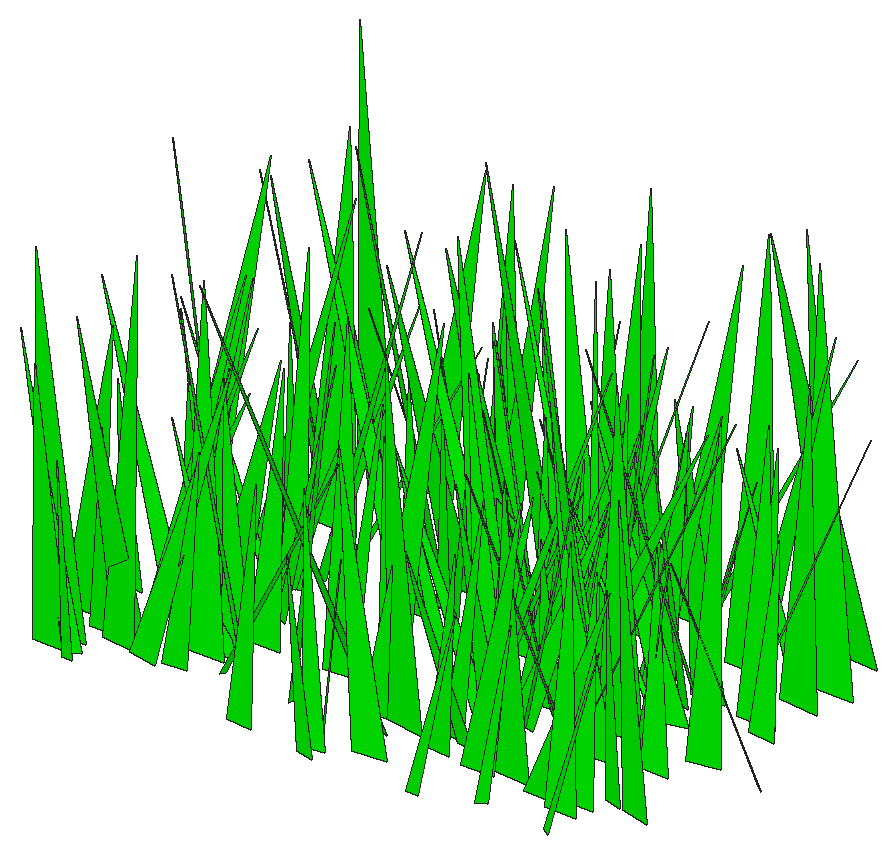
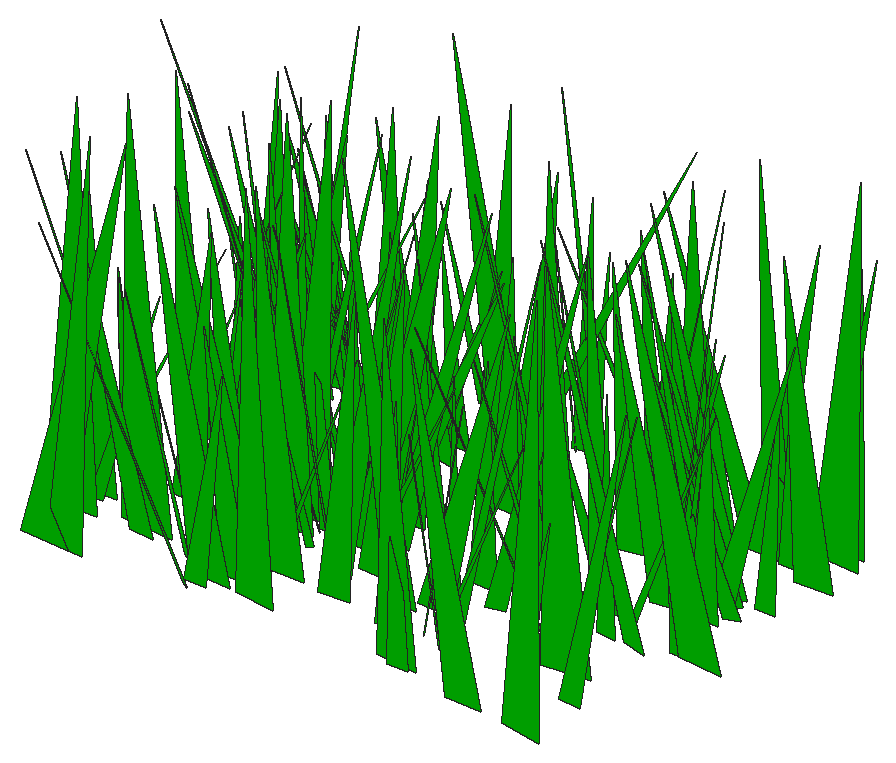
# SketchUp Ruby script. Lengths in inches.
U = 1.inch
M = Sketchup.active_model
def pt(a) = Geom::Point3d.new(a.map { |v| v * U })
def face(e, loops, mat)
  f = e.add_face(loops[0].map { |a| pt(a) })
  loops[1..].each { |l| e.add_face(l.map { |a| pt(a) }).erase! }
  f.material = f.back_material = mat if mat
  f
end
# faces: each face lists its corners as indices into pts; further lists are holes
def faces(e, pts, list, mat = nil) = list.each { |f| face(e, (f[0].is_a?(Array) ? f : [f]).map { |l| l.map { |i| pts[i] } }, mat) }
# xy, xz, yz: faces in a plane at the given z, y or x. An outline is a flat list of corners, or four numbers for a rectangle; further outlines are holes
def ring(l) = l.size == 4 ? [[l[0], l[1]], [l[2], l[1]], [l[2], l[3]], [l[0], l[3]]] : l.each_slice(2).to_a
def flat(e, list, mat, &to3) = list.each { |f| face(e, (f[0].is_a?(Array) ? f : [f]).map { |l| ring(l).map { |u, v| to3.(u, v) } }, mat) }
def xy(e, z, list, mat = nil) = flat(e, list, mat) { |x, y| [x, y, z] }
def xz(e, y, list, mat = nil) = flat(e, list, mat) { |x, z| [x, y, z] }
def yz(e, x, list, mat = nil) = flat(e, list, mat) { |y, z| [x, y, z] }
def lines(e, pts, list) = list.each { |a, b| e.add_line(pt(pts[a]), pt(pts[b])) }
# prism: a flat outline (further loops are holes) pulled along v
def prism(e, loops, v, mat = nil)
  f = face(e, loops, mat); d = Geom::Vector3d.new(v.map { |x| x * U })
  f.pushpull(f.normal.samedirection?(d) ? d.length : -d.length)
end
def box(e, o, s, mat = nil) = prism(e, [[o, [o[0] + s[0], o[1], o[2]], [o[0] + s[0], o[1] + s[1], o[2]], [o[0], o[1] + s[1], o[2]]]], [0, 0, s[2]], mat)
def at(x, y, z, deg = 0) = Geom::Transformation.translation(pt([x, y, z])) * Geom::Transformation.rotation(ORIGIN, Z_AXIS, deg.degrees)
def axes(o, x, y, z) = Geom::Transformation.new([*x, 0, *y, 0, *z, 0, *pt(o).to_a, 1])
def part(name) = M.definitions.add(name)
# library, detail: a bought-in or finely detailed component or shape, given as its bounding box
def library(name, o, s) = part(name).tap { |d| box(d.entities, o, s) }
def detail(e, o, s) = box(e.add_group.entities, o, s)
def put(e, d, t, mat = nil) = e.add_instance(d, t).tap { |i| i.material = mat if mat }
def group(e, t, mat = nil) = e.add_group.tap { |g| g.transformation = t; g.material = mat if mat }.entities
root = M.entities
M.materials.add("[0065_Lime]").color = [0, 255, 0]
c1 = part("fur_instance\#9")
p = [[0.8125,0,1.79],[0.67,-0.02,1.48],[0,-0.11,0],[0,0.11,0]]
faces(c1.entities,p,[[0,1,2,3]])
put(root,c1,axes([66.16,23.27,1.48],[-2.25498,-0.5227,0.91359],[3.79834,-0.33499,-0.21919],[0.81912,0.11443,3.53148]),"[0065_Lime]")
put(root,c1,axes([67.46,23.67,1.48],[-5.30338,0.46201,0.91212],[-3.37935,-0.75276,-0.22369],[0.8049,-0.11631,5.07068]),"[0065_Lime]")
put(root,c1,axes([66.42,19.65,1.48],[-0.43219,-1.1096,1.96187],[8.2532,-0.04828,0.28798],[-0.2379,0.34091,6.42628]),"[0065_Lime]")
put(root,c1,axes([67.59,30.83,1.48],[-6.41038,-0.13063,1.23017],[1.0527,-0.92088,0.35288],[1.4294,0.09238,5.257]),"[0065_Lime]")
put(root,c1,axes([67.24,31.19,1.48],[-4.99882,-0.57823,1.12049],[4.16598,-0.72211,-0.18998],[1.21459,0.09704,5.26315]),"[0065_Lime]")
put(root,c1,axes([67.28,19.06,1.48],[-5.88071,0.31736,1.53233],[-2.48222,-0.85299,-0.38313],[1.57741,-0.15913,5.10975]),"[0065_Lime]")
put(root,c1,axes([66.5,19.01,1.48],[-0.59034,-0.84096,1.06592],[6.12601,-0.08337,0.04076],[0.0776,0.18395,4.8915]),"[0065_Lime]")
put(root,c1,axes([65.95,21.25,1.48],[2.23254,-0.91834,0.53281],[6.56668,0.31413,-0.06238],[-0.13883,0.0906,5.61725]),"[0065_Lime]")
put(root,c1,axes([65.62,27.03,1.48],[4.08051,1.07997,0.77488],[-7.72236,0.57883,-0.12647],[-0.5848,-0.10791,7.07697]),"[0065_Lime]")
put(root,c1,axes([66.42,26.9,1.48],[1.95205,-0.53918,0.17976],[3.82124,0.276,0.28532],[-0.41291,0.00521,3.4902]),"[0065_Lime]")
put(root,c1,axes([67.27,33.47,1.48],[5.46045,0.90805,3.23613],[-7.03555,0.86389,-0.26824],[-2.84417,-0.39364,6.87649]),"[0065_Lime]")
put(root,c1,axes([67.94,25.54,1.48],[-8.50524,-0.12042,2.24811],[0.81591,-1.25665,-0.21315],[2.7762,0.00041,6.95004]),"[0065_Lime]")
put(root,c1,axes([68.75,26.39,1.48],[-5.34362,0.09829,0.51648],[-0.72094,-0.75548,-0.11765],[0.61046,-0.03187,4.38207]),"[0065_Lime]")
put(root,c1,axes([67.375,18.69,1.48],[-3.30569,-0.2481,1.3573],[2.08591,-0.49283,0.34268],[1.24527,0.16692,3.02907]),"[0065_Lime]")
put(root,c1,axes([67.18,20.69,1.48],[0.57871,-0.67566,0.21455],[4.81471,0.08189,0.04845],[-0.09074,0.03579,3.93909]),"[0065_Lime]")
put(root,c1,axes([67.29,24.75,1.48],[1.22999,-0.65895,0.25851],[4.68118,0.17589,0.28718],[-0.42265,0.03047,3.93303]),"[0065_Lime]")
put(root,c1,axes([68.31,20.53,1.48],[-3.34036,-0.8749,0.67141],[6.24904,-0.47614,-0.22049],[0.63043,0.084,5.74313]),"[0065_Lime]")
put(root,c1,axes([68.48,24.25,1.48],[-5.59399,0.05928,1.47973],[-0.39154,-0.82656,0.13027],[1.82593,0.00438,4.56128]),"[0065_Lime]")
put(root,c1,axes([68.44,32.16,1.48],[-1.62054,-0.51068,0.87539],[3.78886,-0.22271,0.28716],[0.10254,0.1585,3.22396]),"[0065_Lime]")
put(root,c1,axes([68.02,20.32,1.48],[5.42273,0.80374,2.29699],[-6.00528,0.81886,-0.22097],[-2.15112,-0.25989,6.40733]),"[0065_Lime]")
put(root,c1,axes([66.66,24.23,1.48],[4.40489,-0.36822,0.18728],[2.62842,0.61863,-0.14644],[-0.10561,0.03829,4.1665]),"[0065_Lime]")
put(root,c1,axes([67.51,24.43,1.48],[6.80886,-0.23616,1.41695],[1.6942,0.98689,0.12509],[-1.72878,0.03703,5.70327]),"[0065_Lime]")
put(root,c1,axes([68.51,29.78,1.48],[-1.07402,1.13371,2.28868],[-8.50769,-0.17891,0.32817],[0.79397,-0.38352,6.61246]),"[0065_Lime]")
put(root,c1,axes([66.97,23.53,1.48],[6.60498,-0.13568,0.73779],[0.99165,0.93611,-0.1052],[-0.87844,0.03658,5.42866]),"[0065_Lime]")
put(root,c1,axes([68.96,27.32,1.48],[-3.51161,-0.44272,1.63919],[3.3832,-0.5416,-0.10625],[1.59424,0.17418,3.83609]),"[0065_Lime]")
put(root,c1,axes([67.28,23.22,1.48],[7.21446,-0.38154,1.2677],[2.80439,1.03212,-0.15033],[-1.39178,0.10191,6.2684]),"[0065_Lime]")
put(root,c1,axes([67.84,27.39,1.48],[7.08674,0.59381,1.14218],[-4.21722,1.01405,-0.35304],[-1.42985,-0.04778,6.70221]),"[0065_Lime]")
put(root,c1,axes([68.67,24.8125,1.48],[2.56931,-0.75627,0.29133],[5.39257,0.35891,-0.2462],[0.11954,0.06372,4.8448]),"[0065_Lime]")
put(root,c1,axes([71.04,21.74,1.48],[-3.82043,0.38239,0.51024],[-2.75701,-0.54023,-0.09168],[0.4448,-0.06414,3.81425]),"[0065_Lime]")
put(root,c1,axes([70.36,21.38,1.48],[-3.24739,0.95358,1.95404],[-7.06678,-0.49287,0.28926],[1.37252,-0.28151,6.11259]),"[0065_Lime]")
put(root,c1,axes([70.02,21.92,1.48],[1.85811,0.7406,0.9841],[-5.37903,0.27159,-0.12898],[-0.55511,-0.15269,4.5439]),"[0065_Lime]")
put(root,c1,axes([69.97,26.18,1.48],[5.60551,-0.59461,2.05984],[4.4352,0.8434,0.17239],[-2.15593,0.18903,5.71031]),"[0065_Lime]")
put(root,c1,axes([71.84,21.46,1.48],[-7.65862,-0.05781,1.60611],[0.39395,-1.11136,-0.09762],[1.97809,-0.00251,6.23784]),"[0065_Lime]")
put(root,c1,axes([69.71,33.16,1.48],[3.4175,0.87898,1.44837],[-6.47866,0.4849,0.25349],[-0.57101,-0.24101,5.79243]),"[0065_Lime]")
put(root,c1,axes([69.06,29.27,1.48],[5.48476,0.34359,0.58273],[-2.43652,0.77716,-0.18124],[-0.74524,-0.01216,4.88128]),"[0065_Lime]")
put(root,c1,axes([69.1,20.1,1.48],[5.21406,0.67149,0.79556],[-4.8413,0.73697,0.14988],[-0.5951,-0.1121,5.75103]),"[0065_Lime]")
put(root,c1,axes([70.16,20.29,1.48],[-2.53264,0.44344,2.28858],[-3.84939,-0.43244,-0.01078],[1.74842,-0.30975,3.29134]),"[0065_Lime]")
put(root,c1,axes([72.53,28.1,1.48],[-7.96476,0.35427,1.50228],[-2.66171,-1.14128,-0.31841],[1.63785,-0.13194,6.788]),"[0065_Lime]")
put(root,c1,axes([71.32,21.82,1.48],[-3.07486,0.63298,1.66726],[-4.82978,-0.45779,-0.06949],[1.08006,-0.24509,4.43586]),"[0065_Lime]")
put(root,c1,axes([69.8,26.12,1.48],[3.59393,-0.3414,0.28709],[2.44313,0.506,-0.0728],[-0.24204,0.03822,3.52793]),"[0065_Lime]")
put(root,c1,axes([72.74,29.57,1.48],[-7.98358,-0.31578,1.68144],[2.38952,-1.15235,0.25487],[1.9009,0.12233,6.7415]),"[0065_Lime]")
put(root,c1,axes([72.84,30.26,1.48],[-4.9798,-0.15271,0.37572],[1.0649,-0.70232,-0.22704],[0.51036,-0.02466,4.13976]),"[0065_Lime]")
put(root,c1,axes([71.48,22.89,1.48],[-2.76944,0.67088,2.02845],[-5.12736,-0.44906,0.345],[1.65017,-0.2694,4.47629]),"[0065_Lime]")
put(root,c1,axes([70.85,24.49,1.48],[5.4425,0.26259,1.24899],[-2.03068,0.78471,0.32637],[-1.31387,-0.12509,4.6693]),"[0065_Lime]")
put(root,c1,axes([70.32,27.08,1.48],[8.24277,-0.07571,1.35435],[0.61659,1.17996,-0.27254],[-1.63781,0.06317,6.71355]),"[0065_Lime]")
put(root,c1,axes([73.22,30.64,1.48],[-4.96317,-0.08246,1.16918],[0.53454,-0.72592,-0.21431],[1.45764,-0.01457,4.05957]),"[0065_Lime]")
put(root,c1,axes([72.59,32.67,1.48],[3.76043,-0.44685,1.31627],[3.22968,0.5667,0.3418],[-1.51672,0.09883,3.99128]),"[0065_Lime]")
put(root,c1,axes([73.91,29.25,1.48],[-3.65675,-0.86088,0.18332],[6.11872,-0.51479,-0.25244],[0.38202,0.00481,5.79806]),"[0065_Lime]")
put(root,c1,axes([70.44,28.46,1.48],[5.97385,0.17399,0.03922],[-1.23556,0.83891,-0.18811],[-0.09412,0.03045,4.95892]),"[0065_Lime]")
put(root,c1,axes([72.78,32.46,1.48],[2.54539,0.96582,1.46261],[-7.02446,0.38232,-0.37134],[-1.06405,-0.21354,5.95031]),"[0065_Lime]")
put(root,c1,axes([72.4375,30.89,1.48],[4.13364,0.09899,1.01993],[-0.6079,0.60618,-0.3414],[-1.30346,0.03123,3.39371]),"[0065_Lime]")
put(root,c1,axes([72.47,25.91,1.48],[4.22336,-0.32963,0.95726],[2.32756,0.61519,0.30415],[-1.21258,0.03278,3.91791]),"[0065_Lime]")
put(root,c1,axes([73.69,27.25,1.48],[0.05595,0.63866,1.42593],[-4.86831,0.01612,-0.1156],[-0.17387,-0.24593,3.69549]),"[0065_Lime]")
put(root,c1,axes([71.53,20.88,1.48],[5.81626,-0.04275,0.16488],[0.31121,0.81725,-0.16263],[-0.19185,0.02956,4.7347]),"[0065_Lime]")
put(root,c1,axes([77.32,21.14,1.48],[-8.29368,-0.43806,0.05103],[3.1169,-1.16542,-0.0673],[0.08783,-0.00778,7.20672]),"[0065_Lime]")
put(root,c1,axes([73.81,18.8,1.48],[2.46524,0.60398,1.27183],[-4.49646,0.36574,-0.05349],[-0.83766,-0.18575,4.03015]),"[0065_Lime]")
put(root,c1,axes([74.22,27.97,1.48],[3.37891,0.32692,1.55955],[-2.60392,0.52042,0.07711],[-1.51939,-0.16486,3.33608]),"[0065_Lime]")
put(root,c1,axes([74.34,30.9,1.48],[-1.22104,-0.66221,0.48853],[4.71481,-0.17961,-0.3614],[0.58337,0.06558,3.94338]),"[0065_Lime]")
put(root,c1,axes([74.33,23,1.48],[4.62307,-0.74048,2.53866],[5.80371,0.70518,-0.10046],[-1.95629,0.34215,5.70126]),"[0065_Lime]")
put(root,c1,axes([74.18,20.83,1.48],[7.97859,-0.00673,2.21488],[0.07072,1.18457,-0.04802],[-2.72244,0.01106,6.48983]),"[0065_Lime]")
put(root,c1,axes([77.12,27.05,1.48],[-7.5152,0.46836,1.07464],[-3.35559,-1.07066,0.10974],[1.26293,-0.0577,6.68631]),"[0065_Lime]")
put(root,c1,axes([76.65,25.0625,1.48],[-3.39333,0.39063,0.33505],[-2.7841,-0.47963,0.08172],[0.3825,-0.0257,3.56721]),"[0065_Lime]")
put(root,c1,axes([77.23,28.31,1.48],[-4.42247,-0.22079,0.16243],[1.56722,-0.62203,-0.09987],[0.22924,-0.00688,3.81629]),"[0065_Lime]")
put(root,c1,axes([74.93,29.59,1.48],[6.57719,0.82445,2.0909],[-6.13059,0.96026,0.07179],[-1.85691,-0.25008,7.16895]),"[0065_Lime]")
put(root,c1,axes([76.0625,23.26,1.48],[-2.5226,0.5618,2.12879],[-4.66767,-0.37874,-0.31041],[1.02308,-0.34271,3.83276]),"[0065_Lime]")
put(root,c1,axes([76.76,28.51,1.48],[1.82538,0.39521,1.93727],[-3.27487,0.34524,-0.31838],[-1.69046,-0.24207,2.70868]),"[0065_Lime]")
put(root,c1,axes([76.49,28.72,1.48],[0.10413,-0.88897,1.15129],[6.4683,0.02754,0.32551],[-0.43325,0.19751,5.13637]),"[0065_Lime]")
put(root,c1,axes([76.5,18.52,1.48],[2.57943,0.35227,1.77473],[-2.9717,0.41823,0.07598],[-1.48795,-0.22461,2.92482]),"[0065_Lime]")
put(root,c1,axes([76.73,30.52,1.48],[3.7401,-0.63238,2.62586],[5.08722,0.60865,0.11757],[-2.18965,0.33394,4.75833]),"[0065_Lime]")
put(root,c1,axes([75.76,26.45,1.48],[5.41329,0.23496,1.69926],[-1.92134,0.80238,0.33199],[-1.86242,-0.14481,4.59655]),"[0065_Lime]")
put(root,c1,axes([77.62,29.17,1.48],[-7.66387,-0.68354,2.15937],[5.17113,-1.11098,0.35878],[1.99242,0.25419,7.37489]),"[0065_Lime]")
put(root,c1,axes([76.51,18.97,1.48],[-4.0421,0.42616,1.69238],[-3.301,-0.61192,-0.05316],[1.62169,-0.18339,4.1101]),"[0065_Lime]")
put(root,c1,axes([77.6,27.71,1.48],[-3.2373,-1.10351,0.73996],[7.90555,-0.45262,0.26547],[0.04299,0.13567,6.90423]),"[0065_Lime]")
put(root,c1,axes([77.66,27.26,1.48],[-1.34589,0.87733,0.8543],[-6.33014,-0.18362,-0.27947],[-0.11938,-0.15437,5.18772]),"[0065_Lime]")
put(root,c1,axes([76.67,19.12,1.48],[3.93671,0.07634,1.14014],[-0.61335,0.58564,0.08723],[-1.37246,-0.04275,3.23135]),"[0065_Lime]")
put(root,c1,axes([78.03,25.67,1.48],[4.01712,-0.93613,3.79121],[7.66995,0.67871,0.23857],[-2.69783,0.53565,6.32342]),"[0065_Lime]")
put(root,c1,axes([78.05,19.69,1.48],[-2.72319,0.78572,1.00962],[-5.71206,-0.38682,-0.1063],[0.42353,-0.16497,5.05791]),"[0065_Lime]")
put(root,c1,axes([79.26,23.5625,1.48],[-4.63226,0.38736,0.27369],[-2.77518,-0.64911,-0.29286],[0.10402,-0.06768,4.37488]),"[0065_Lime]")
put(root,c1,axes([77.77,21.7,1.48],[-4.21866,-0.8743,2.02721],[6.5031,-0.63411,-0.21],[1.62292,0.26824,6.11108]),"[0065_Lime]")
put(root,c1,axes([76.88,21.75,1.48],[6.48516,-0.81641,2.03136],[6.1259,0.93581,-0.33675],[-1.57054,0.27897,7.07448]),"[0065_Lime]")
put(root,c1,axes([77.26,29.78,1.48],[6.6487,0.06247,1.44561],[-0.53434,0.96536,0.22806],[-1.75233,-0.05733,5.41542]),"[0065_Lime]")
put(root,c1,axes([79.84,28.91,1.48],[-4.52867,-0.14205,0.4692],[1.00661,-0.64149,-0.07962],[0.58433,0.00413,3.7735]),"[0065_Lime]")
put(root,c1,axes([78.42,32.15,1.48],[4.91072,0.91486,2.59144],[-6.93859,0.74971,-0.16928],[-2.09622,-0.33838,6.63119]),"[0065_Lime]")
put(root,c1,axes([79.17,24.06,1.48],[-4.43021,0.70785,1.47417],[-5.16622,-0.65195,0.21745],[1.40384,-0.16538,5.45238]),"[0065_Lime]")
put(root,c1,axes([79.9,21.92,1.48],[-3.60664,-0.40353,0.25717],[2.87662,-0.50817,-0.02702],[0.26807,0.02401,3.74996]),"[0065_Lime]")
put(root,c1,axes([78.02,25.36,1.48],[2.03339,0.55065,0.20938],[-3.92447,0.28643,-0.0253],[-0.14621,-0.03009,3.59104]),"[0065_Lime]")
put(root,c1,axes([80.76,27.11,1.48],[-8.59443,0.18782,1.67238],[-1.30147,-1.24175,0.2477],[2.07842,-0.00092,7.07052]),"[0065_Lime]")
put(root,c1,axes([78.84,30.39,1.48],[1.62357,1.09053,1.87653],[-8.08841,0.23316,0.08979],[-0.35983,-0.32058,6.44875]),"[0065_Lime]")
put(root,c1,axes([79.87,23.25,1.48],[1.95957,0.51226,2.3944],[-4.41287,0.35249,-0.13747],[-1.57523,-0.35023,3.36374]),"[0065_Lime]")
put(root,c1,axes([80.76,25.01,1.48],[-5.84517,-0.13162,0.98087],[1.00278,-0.83647,0.19258],[1.1515,0.06031,4.81135]),"[0065_Lime]")
put(root,c1,axes([79.62,25.9,1.48],[4.38715,-0.41316,2.04313],[3.34835,0.67289,-0.19744],[-1.93469,0.22767,4.29136]),"[0065_Lime]")
put(root,c1,axes([79.37,27.5,1.48],[3.84037,-0.32574,1.11618],[2.32705,0.5703,0.27963],[-1.3571,0.05611,3.63807]),"[0065_Lime]")
put(root,c1,axes([79.45,21.17,1.48],[1.80793,0.52024,1.0333],[-3.88081,0.26387,0.0409],[-0.5101,-0.16363,3.35115]),"[0065_Lime]")
put(root,c1,axes([80.3125,27.28,1.48],[-5.8365,0.95902,2.11109],[-7.02369,-0.865,0.31933],[1.99574,-0.23958,7.29763]),"[0065_Lime]")
put(root,c1,axes([79.27,22.125,1.48],[3.49375,0.53621,0.93835],[-3.84058,0.51051,-0.31428],[-1.0688,-0.08166,4.19666]),"[0065_Lime]")
put(root,c1,axes([79.29,25.68,1.48],[-2.13128,-0.37525,1.95702],[3.22751,-0.37279,-0.06962],[1.58213,0.25498,2.77831]),"[0065_Lime]")
put(root,c1,axes([78.35,25.35,1.48],[5.02938,-0.07147,0.43522],[0.55457,0.70749,-0.34733],[-0.48724,0.06757,4.09713]),"[0065_Lime]")
put(root,c1,axes([80.45,32.43,1.48],[-2.23561,-0.55522,0.71715],[4.00869,-0.32338,-0.12115],[0.56598,0.09727,3.69081]),"[0065_Lime]")
put(root,c1,axes([79.2,28.56,1.48],[4.13858,-0.13167,0.66632],[0.97318,0.5915,-0.08254],[-0.7759,0.03957,3.4506]),"[0065_Lime]")
put(root,c1,axes([80.21,23.11,1.48],[0.78263,0.72462,0.65026],[-5.20539,0.11642,-0.20194],[-0.36813,-0.10564,4.23783]),"[0065_Lime]")
put(root,c1,axes([78.53,26.83,1.48],[5.58678,0.29292,0.67329],[-2.14894,0.78848,0.30314],[-0.64246,-0.09011,4.84092]),"[0065_Lime]")
put(root,c1,axes([79.68,31.49,1.48],[1.41785,-0.69003,0.62959],[4.96823,0.19272,-0.32487],[0.17404,0.11992,4.14484]),"[0065_Lime]")
put(root,c1,axes([80.48,25.26,1.48],[0.35631,-0.56953,0.03809],[4.04973,0.0503,0.13694],[-0.17182,0.00448,3.30673]),"[0065_Lime]")
put(root,c1,axes([80.43,28.03,1.48],[-1.60427,-1.13229,2.36148],[8.52211,-0.2525,-0.22635],[0.856,0.39177,6.67925]),"[0065_Lime]")
put(root,c1,axes([82.02,25.99,1.48],[-4.73134,-0.05517,0.54403],[0.4032,-0.67129,0.03893],[0.66251,0.01454,3.86157]),"[0065_Lime]")
put(root,c1,axes([80.65,27.01,1.48],[7.88385,-0.20301,2.81265],[1.42115,1.20921,0.28897],[-3.4676,0.03402,6.51321]),"[0065_Lime]")
put(root,c1,axes([80.26,31.98,1.48],[3.50132,1.00616,0.98075],[-7.2314,0.5002,-0.11411],[-0.65703,-0.14342,6.48238]),"[0065_Lime]")
put(root,c1,axes([80.43,18.71,1.48],[3.39261,0.34448,0.55244],[-2.44308,0.48555,-0.2186],[-0.70881,-0.02477,3.39763]),"[0065_Lime]")
put(root,c1,axes([78.85,24.19,1.48],[8.03495,0.31835,0.9196],[-2.31868,1.13749,0.20935],[-1.01711,-0.07822,6.78734]),"[0065_Lime]")
put(root,c1,axes([83.33,26.66,1.48],[-5.2668,0.078,0.05052],[-0.5536,-0.73995,0.09893],[0.0745,0.01608,4.30668]),"[0065_Lime]")
put(root,c1,axes([79.92,26.34,1.48],[5.35146,0.49576,0.60922],[-3.50586,0.75923,-0.32714],[-0.84694,-0.01031,5.20355]),"[0065_Lime]")
put(root,c1,axes([80.54,23.91,1.48],[5.65135,0.03052,1.16965],[-0.12667,0.81804,-0.31043],[-1.44874,0.04755,4.58979]),"[0065_Lime]")
put(root,c1,axes([80.375,27.05,1.48],[5.58269,0.76138,1.23649],[-5.54728,0.79517,0.16417],[-0.94724,-0.16946,6.32606]),"[0065_Lime]")
put(root,c1,axes([80.37,23.99,1.48],[3.58335,0.61364,0.29795],[-4.38201,0.50088,0.30193],[0.0557,-0.07286,4.58505]),"[0065_Lime]")
put(root,c1,axes([81.09,21.01,1.48],[3.43681,-0.71818,1.07343],[5.25343,0.48695,-0.21167],[-0.51488,0.17461,5.00537]),"[0065_Lime]")
put(root,c1,axes([84.25,22.125,1.48],[-6.04465,-0.15488,0.23101],[1.10816,-0.85003,0.08837],[0.25984,0.02219,4.99709]),"[0065_Lime]")
put(root,c1,axes([83.06,24.09,1.48],[-8.13868,-0.5413,2.35865],[4.0961,-1.19794,0.13924],[2.54353,0.19713,7.3229]),"[0065_Lime]")
put(root,c1,axes([79.63,27.6,1.48],[8.62317,0.18401,0.97662],[-1.31131,1.22331,-0.06276],[-1.19868,-0.01451,7.09434]),"[0065_Lime]")
put(root,c1,axes([83.91,26.79,1.48],[-4.18786,0.68031,0.3491],[-4.86032,-0.58557,-0.33884],[-0.03558,-0.08389,5.19595]),"[0065_Lime]")
put(root,c1,axes([82.08,21.28,1.48],[-0.12793,-0.94753,0.70213],[6.79536,-0.02132,-0.14504],[0.19611,0.12075,5.48405]),"[0065_Lime]")
put(root,c1,axes([83.26,23.76,1.48],[-3.14936,0.96212,0.57034],[-6.87821,-0.4439,-0.03711],[0.25137,-0.0922,6.13023]),"[0065_Lime]")
put(root,c1,axes([81.51,26.63,1.48],[7.46528,-0.02312,1.92548],[0.09527,1.10011,0.19827],[-2.37096,-0.0286,6.07059]),"[0065_Lime]")
put(root,c1,axes([81.59,24.19,1.48],[4.68342,0.27242,1.00683],[-1.99861,0.67727,0.01061],[-1.13853,-0.06827,4.12303]),"[0065_Lime]")
put(root,c1,axes([82.22,25.96,1.48],[6.00421,-0.36362,2.11674],[2.80389,0.9069,-0.04185],[-2.3678,0.15187,5.31802]),"[0065_Lime]")
put(root,c1,axes([83.06,27.25,1.48],[-3.00898,-0.64269,1.06038],[4.66659,-0.44079,-0.19072],[0.91718,0.13428,4.44914]),"[0065_Lime]")
put(root,c1,axes([81.61,31.36,1.48],[5.15648,0.19769,0.8433],[-1.34341,0.73868,-0.36758],[-1.11777,0.02419,4.33209]),"[0065_Lime]")
put(root,c1,axes([83.47,27.83,1.48],[4.36631,0.23172,2.28131],[-1.90239,0.71691,-0.03097],[-2.63934,-0.1334,3.79634]),"[0065_Lime]")
put(root,c1,axes([82.21,28.18,1.48],[3.29132,-0.70053,1.18635],[5.14291,0.47355,-0.07037],[-0.72915,0.17791,4.8587]),"[0065_Lime]")
put(root,c1,axes([82.42,19.53,1.48],[3.61723,-0.26089,0.77534],[1.85676,0.52466,0.18426],[-0.95294,0.03198,3.30211]),"[0065_Lime]")
put(root,c1,axes([82.0625,30.4,1.48],[4.17669,0.10015,0.60798],[-0.69923,0.59622,-0.11282],[-0.76009,0.00185,3.44464]),"[0065_Lime]")
put(root,c1,axes([83.12,25.25,1.48],[1.91261,-1.01141,1.59482],[7.41929,0.28756,0.22381],[-0.77816,0.25582,6.05376]),"[0065_Lime]")
put(root,c1,axes([81.76,28.35,1.48],[5.31352,-0.51379,0.94439],[3.75239,0.75404,-0.22255],[-0.798,0.12458,5.24181]),"[0065_Lime]")
put(root,c1,axes([80.64,32.69,1.48],[6.97502,0.20566,0.12729],[-1.46595,0.98019,0.08142],[-0.13258,-0.01829,5.79656]),"[0065_Lime]")
put(root,c1,axes([80.69,25.94,1.48],[6.82757,-0.44017,0.1875],[3.13995,0.95846,-0.253],[-0.07956,0.05324,6.10501]),"[0065_Lime]")
put(root,c1,axes([83.76,28.59,1.48],[-0.13042,-0.80534,0.87884],[5.82748,-0.01188,0.20746],[-0.23491,0.15246,4.65848]),"[0065_Lime]")
put(root,c1,axes([86.26,25.84,1.48],[-8.01336,-0.11415,0.74838],[0.80083,-1.13339,-0.11942],[0.93011,-0.00762,6.55049]),"[0065_Lime]")
put(root,c1,axes([83.66,30.73,1.48],[2.69074,1.21557,1.9993],[-8.93663,0.40174,-0.22711],[-1.00592,-0.31756,7.36559]),"[0065_Lime]")
put(root,c1,axes([85.59,33.18,1.48],[-3.7191,-1.19696,0.54023],[8.53851,-0.52436,-0.03846],[0.30918,0.08286,7.56037]),"[0065_Lime]")
put(root,c1,axes([84.79,33.22,1.48],[-5.53082,-0.90384,2.24168],[6.67707,-0.82934,-0.305],[2.09397,0.25722,6.89352]),"[0065_Lime]")
put(root,c1,axes([84.31,30.49,1.48],[-3.07131,0.48831,1.63389],[-3.64663,-0.48797,0.35148],[1.67727,-0.16675,3.75605]),"[0065_Lime]")
put(root,c1,axes([84.59,20.55,1.48],[-2.56714,0.67199,1.63391],[-5.01275,-0.40235,0.33398],[1.33308,-0.21888,4.40233]),"[0065_Lime]")
put(root,c1,axes([85.97,30.24,1.48],[-4.57139,0.25437,0.71121],[-1.88377,-0.64859,-0.23799],[0.70208,-0.08398,3.99228]),"[0065_Lime]")
put(root,c1,axes([84.78,21.18,1.48],[1.14738,0.71261,0.35912],[-5.07846,0.16461,-0.2096],[-0.34954,-0.05242,4.22412]),"[0065_Lime]")
put(root,c1,axes([83.45,20.91,1.48],[3.358,-0.61081,0.16536],[4.34803,0.4695,-0.3082],[0.17606,0.05512,4.4573]),"[0065_Lime]")
put(root,c1,axes([83.55,31.12,1.48],[6.10369,0.61948,1.40187],[-4.5907,0.87103,0.32692],[-1.15372,-0.18856,6.1157]),"[0065_Lime]")
put(root,c1,axes([84.46,24.31,1.48],[3.97918,0.20703,0.9349],[-1.45466,0.58169,-0.21982],[-1.17287,-0.01907,3.44444]),"[0065_Lime]")
put(root,c1,axes([85.28,24.15,1.48],[-1.68397,0.63412,0.50747],[-4.51103,-0.24515,0.36052],[0.63591,-0.05983,3.90132]),"[0065_Lime]")
put(root,c1,axes([82.33,24.25,1.48],[8.5429,0.06906,0.46711],[-0.49362,1.20312,0.01306],[-0.57239,-0.00689,6.96039]),"[0065_Lime]")
put(root,c1,axes([85.5,21.91,1.48],[3.31896,0.32309,1.72234],[-2.69169,0.51605,0.18803],[-1.58904,-0.19931,3.27885]),"[0065_Lime]")
put(root,c1,axes([85.77,28.36,1.48],[-1.26177,0.85656,1.2682],[-6.25271,-0.19563,0.31148],[0.70199,-0.20289,5.05389]),"[0065_Lime]")
put(root,c1,axes([86.22,31.14,1.48],[-1.78822,1.18167,2.16415],[-8.80419,-0.26214,-0.01711],[0.53185,-0.36633,6.99324]),"[0065_Lime]")
put(root,c1,axes([84.97,19.39,1.48],[4.12592,0.15431,0.68941],[-1.17176,0.58771,0.23199],[-0.74243,-0.07005,3.46515]),"[0065_Lime]")
put(root,c1,axes([86.5,21.72,1.48],[-4.46988,-0.63404,1.75408],[4.68119,-0.67347,-0.26463],[1.75972,0.18101,5.1595]),"[0065_Lime]")
put(root,c1,axes([86.11,29.95,1.48],[-1.70499,-0.85243,2.22006],[6.56992,-0.2778,-0.23588],[1.04193,0.3568,5.12019]),"[0065_Lime]")
put(root,c1,axes([86.12,25.43,1.48],[-4.58132,0.65286,3.09671],[-5.44654,-0.73521,-0.13743],[2.53285,-0.40009,5.3057]),"[0065_Lime]")
put(root,c1,axes([86.42,27.81,1.48],[-0.16594,0.61242,0.37341],[-4.37332,-0.0273,0.21449],[0.28239,-0.06292,3.54119]),"[0065_Lime]")
put(root,c1,axes([88.35,25.33,1.48],[-4.36715,-0.11739,0.11822],[0.83699,-0.61394,0.02921],[0.136,0.0088,3.61659]),"[0065_Lime]")
put(root,c1,axes([84.71,29.51,1.48],[6.8145,0.09165,0.48872],[-0.68838,0.95915,0.3236],[-0.55903,-0.06389,5.55892]),"[0065_Lime]")
